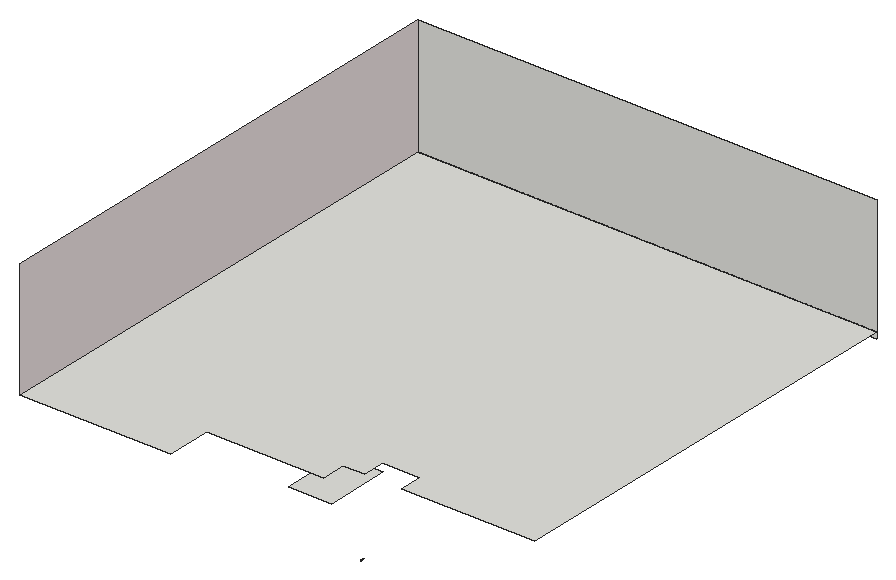
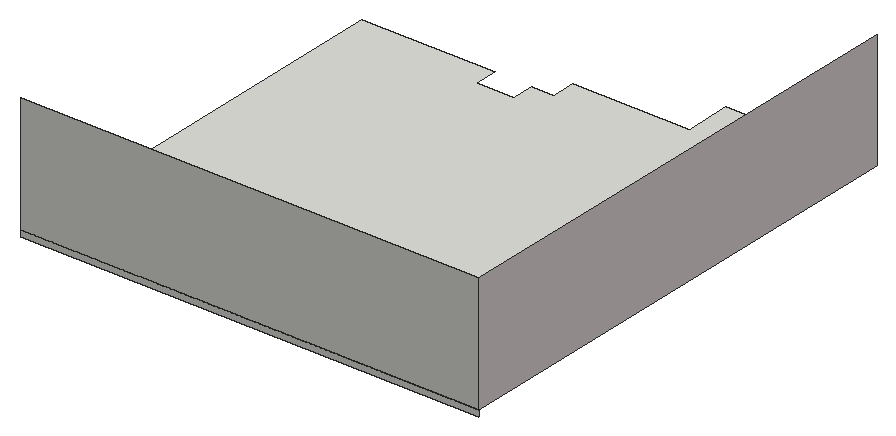
# SketchUp Ruby script. Lengths in inches.
U = 1.inch
M = Sketchup.active_model
def pt(a) = Geom::Point3d.new(a.map { |v| v * U })
def face(e, loops, mat)
  f = e.add_face(loops[0].map { |a| pt(a) })
  loops[1..].each { |l| e.add_face(l.map { |a| pt(a) }).erase! }
  f.material = f.back_material = mat if mat
  f
end
# faces: each face lists its corners as indices into pts; further lists are holes
def faces(e, pts, list, mat = nil) = list.each { |f| face(e, (f[0].is_a?(Array) ? f : [f]).map { |l| l.map { |i| pts[i] } }, mat) }
# xy, xz, yz: faces in a plane at the given z, y or x. An outline is a flat list of corners, or four numbers for a rectangle; further outlines are holes
def ring(l) = l.size == 4 ? [[l[0], l[1]], [l[2], l[1]], [l[2], l[3]], [l[0], l[3]]] : l.each_slice(2).to_a
def flat(e, list, mat, &to3) = list.each { |f| face(e, (f[0].is_a?(Array) ? f : [f]).map { |l| ring(l).map { |u, v| to3.(u, v) } }, mat) }
def xy(e, z, list, mat = nil) = flat(e, list, mat) { |x, y| [x, y, z] }
def xz(e, y, list, mat = nil) = flat(e, list, mat) { |x, z| [x, y, z] }
def yz(e, x, list, mat = nil) = flat(e, list, mat) { |y, z| [x, y, z] }
def lines(e, pts, list) = list.each { |a, b| e.add_line(pt(pts[a]), pt(pts[b])) }
# prism: a flat outline (further loops are holes) pulled along v
def prism(e, loops, v, mat = nil)
  f = face(e, loops, mat); d = Geom::Vector3d.new(v.map { |x| x * U })
  f.pushpull(f.normal.samedirection?(d) ? d.length : -d.length)
end
def box(e, o, s, mat = nil) = prism(e, [[o, [o[0] + s[0], o[1], o[2]], [o[0] + s[0], o[1] + s[1], o[2]], [o[0], o[1] + s[1], o[2]]]], [0, 0, s[2]], mat)
def at(x, y, z, deg = 0) = Geom::Transformation.translation(pt([x, y, z])) * Geom::Transformation.rotation(ORIGIN, Z_AXIS, deg.degrees)
def axes(o, x, y, z) = Geom::Transformation.new([*x, 0, *y, 0, *z, 0, *pt(o).to_a, 1])
def part(name) = M.definitions.add(name)
# library, detail: a bought-in or finely detailed component or shape, given as its bounding box
def library(name, o, s) = part(name).tap { |d| box(d.entities, o, s) }
def detail(e, o, s) = box(e.add_group.entities, o, s)
def put(e, d, t, mat = nil) = e.add_instance(d, t).tap { |i| i.material = mat if mat }
def group(e, t, mat = nil) = e.add_group.tap { |g| g.transformation = t; g.material = mat if mat }.entities
root = M.entities
M.materials.add("Generic\#9").color = [233, 223, 223]
M.materials.add("Material \#1").color = [140, 140, 140]
xy(root,89.4,[[280.76,194.8125,322.26,256.5625]])
xy(root,126,[[75.375,127.4375,220.54,127.4375,220.54,171.4375,333.65,171.4375,333.65,194.75,354.24,194.75,354.24,216.25,390.67,216.25,390.67,194.75,518.6875,194.75,518.6875,607.4375,75.375,607.4375]])
xz(root,199.31,[[347.11,46.74,347.11,46.88,347.12,46.875],[347.82,46.79,347.78,46.8,347.82,46.81],[347.82,46.79,347.82,46.81,347.86,46.8125],[347.82,46.79,347.86,46.8125,347.87,46.8],[347.78,46.8,347.74,46.81,347.78,46.8125],
  [347.78,46.8,347.78,46.8125,347.82,46.81],[347.87,46.8,347.86,46.8125,347.9,46.82],[347.87,46.8,347.9,46.82,347.91,46.81],[347.74,46.81,347.7,46.83,347.74,46.82],[347.74,46.81,347.74,46.82,347.78,46.8125],
  [347.12,46.875,347.11,46.88,347.14,47],[347.12,46.875,347.14,47,347.16,47],[347.14,47,347.2,47.12,347.16,47],[347.625,47.16,347.64,47.2,347.65,47.19],[347.65,47.19,347.64,47.2,347.67,47.23],
  [347.65,47.19,347.67,47.23,347.68,47.22],[347.28,47.22,347.36,47.3125,347.36,47.3],[347.68,47.22,347.67,47.23,347.7,47.25],[347.68,47.22,347.7,47.25,347.71,47.24],[347.71,47.24,347.7,47.25,347.74,47.27],
  [347.71,47.24,347.74,47.27,347.74,47.26],[347.74,47.26,347.74,47.27,347.78,47.28],[347.74,47.26,347.78,47.28,347.78,47.27],[347.36,47.3,347.36,47.3125,347.46,47.39],[347.46,47.375,347.46,47.39,347.57,47.44],
  [347.46,47.375,347.57,47.44,347.58,47.43],[347.58,47.43,347.57,47.44,347.69,47.47],[347.58,47.43,347.69,47.47,347.7,47.46],[347.95,47.46,347.82,47.47,347.95,47.47]],"Material \#1")
xz(root,201.11,[[347.1,46.74,347.11,46.74,347.11,46.88],[347.11,46.74,347.12,46.875,347.11,46.88],[347.82,46.79,347.82,46.81,347.78,46.8],[347.82,46.79,347.86,46.8125,347.82,46.81],[347.82,46.79,347.87,46.8,347.86,46.8125],
  [347.78,46.8,347.78,46.8125,347.74,46.81],[347.78,46.8,347.82,46.81,347.78,46.8125],[347.87,46.8,347.9,46.82,347.86,46.8125],[347.87,46.8,347.91,46.81,347.9,46.82],[347.74,46.81,347.74,46.82,347.7,46.83],
  [347.74,46.81,347.78,46.8125,347.74,46.82],[347.91,46.81,347.9375,46.84,347.9,46.82],[347.74,46.82,347.71,46.84,347.7,46.83],[347.7,46.83,347.71,46.84,347.67,46.85],[347.71,46.84,347.68,46.86,347.67,46.85],
  [347.67,46.85,347.68,46.86,347.64,46.88],[347.68,46.86,347.65,46.89,347.64,46.88],[347.12,46.875,347.14,47,347.11,46.88],[347.12,46.875,347.16,47,347.14,47],[347.64,46.88,347.65,46.89,347.62,46.92],
  [347.65,46.89,347.625,46.92,347.62,46.92],[347.62,46.92,347.625,46.92,347.6,46.95],[347.625,46.92,347.61,46.96,347.6,46.95],[347.6,46.95,347.61,46.96,347.59,47],[347.61,46.96,347.6,47,347.59,47],
  [347.14,47,347.16,47,347.2,47.12],[347.16,47,347.21,47.11,347.2,47.12],[347.59,47,347.6,47,347.58,47.05],[347.6,47,347.6,47.05,347.58,47.05],[347.58,47.05,347.6,47.05,347.59,47.09],
  [347.6,47.05,347.6,47.08,347.59,47.09],[347.6,47.08,347.6,47.13,347.59,47.09],[347.6,47.08,347.61,47.12,347.6,47.13],[347.21,47.11,347.27,47.23,347.2,47.12],[347.21,47.11,347.28,47.22,347.27,47.23],
  [347.61,47.12,347.62,47.17,347.6,47.13],[347.61,47.12,347.625,47.16,347.62,47.17],[347.625,47.16,347.64,47.2,347.62,47.17],[347.625,47.16,347.65,47.19,347.64,47.2],[347.65,47.19,347.67,47.23,347.64,47.2],
  [347.65,47.19,347.68,47.22,347.67,47.23],[347.28,47.22,347.36,47.3125,347.27,47.23],[347.28,47.22,347.36,47.3,347.36,47.3125],[347.68,47.22,347.7,47.25,347.67,47.23],[347.68,47.22,347.71,47.24,347.7,47.25],
  [347.71,47.24,347.74,47.27,347.7,47.25],[347.71,47.24,347.74,47.26,347.74,47.27],[347.95,47.25,347.91,47.27,347.9,47.26],[347.74,47.26,347.78,47.27,347.78,47.28],[347.74,47.26,347.78,47.28,347.74,47.27],
  [347.9,47.26,347.91,47.27,347.86,47.27],[347.78,47.27,347.82,47.28,347.82,47.29],[347.78,47.27,347.82,47.29,347.78,47.28],[347.86,47.27,347.87,47.28,347.82,47.28],[347.86,47.27,347.91,47.27,347.87,47.28],
  [347.82,47.28,347.87,47.28,347.82,47.29],[347.36,47.3,347.46,47.375,347.46,47.39],[347.36,47.3,347.46,47.39,347.36,47.3125],[347.46,47.375,347.57,47.44,347.46,47.39],[347.46,47.375,347.58,47.43,347.57,47.44],
  [347.58,47.43,347.69,47.47,347.57,47.44],[347.58,47.43,347.7,47.46,347.69,47.47],[347.7,47.46,347.82,47.49,347.69,47.47],[347.7,47.46,347.82,47.47,347.82,47.49],[347.95,47.46,347.95,47.47,347.82,47.47],
  [347.82,47.47,347.95,47.47,347.82,47.49]],"Material \#1")
xz(root,607.4375,[[75.375,120,518.6875,126],[75.375,126,518.6875,240]])
yz(root,75.375,[[127.4375,126,607.4375,240]],"Generic\#9")
p = [[347.84,199.31,46.96],[347.84,199.33,46.96],[347.85,199.33,46.93],[347.85,199.31,46.93],[347.87,199.34,46.91],[347.87,199.31,46.91],
  [347.89,199.34,46.92],[347.89,199.31,46.92],[347.92,199.34,46.93],[347.92,199.31,46.93],[347.9,199.33,46.96],[347.9,199.31,46.96],
  [347.84,201.12,46.96],[347.85,201.11,46.93],[347.85,201.09,46.93],[347.84,201.09,46.96],[347.87,201.11,46.91],[347.87,201.08,46.91],
  [347.89,201.11,46.92],[347.89,201.08,46.92],[347.92,201.11,46.93],[347.92,201.08,46.93],[347.9,201.11,46.96],[347.9,201.09,46.96],
  [347.76,199.31,47.09],[347.76,199.33,47.09],[347.89,199.31,46.99],[347.89,199.33,46.99],[347.81,199.33,47.125],[347.81,199.31,47.125],
  [347.76,201.12,47.09],[347.76,201.09,47.09],[347.89,201.12,46.99],[347.81,201.12,47.125],[347.81,201.09,47.125],[347.89,201.09,46.99],
  [347.75,199.31,47.17],[347.75,199.34,47.17],[347.73,199.34,47.15],[347.73,199.31,47.15],[347.75,199.33,47.12],[347.75,199.31,47.12],
  [347.8,199.33,47.15],[347.8,199.31,47.15],[347.78,199.34,47.18],[347.78,199.31,47.18],[347.75,201.11,47.17],[347.73,201.11,47.15],
  [347.73,201.08,47.15],[347.75,201.08,47.17],[347.75,201.11,47.12],[347.75,201.09,47.12],[347.8,201.11,47.15],[347.8,201.09,47.15],
  [347.78,201.11,47.18],[347.78,201.08,47.18]]
faces(root,p,[[0,1,2],[2,3,0],[3,2,4],[4,5,3],[5,4,6],[6,7,5],[7,6,8],[8,9,7],
  [9,8,10],[10,11,9],[12,13,14],[14,15,12],[13,16,17],[17,14,13],[16,18,19],[19,17,16],
  [18,20,21],[21,19,18],[20,22,23],[23,21,20],[24,25,1],[1,0,24],[26,27,28],[28,29,26],
  [11,10,27],[27,26,11],[30,12,15],[15,31,30],[32,33,34],[34,35,32],[22,32,35],[35,23,22],
  [36,37,38],[38,39,36],[39,38,40],[40,41,39],[41,40,25],[25,24,41],[29,28,42],[42,43,29],
  [43,42,44],[44,45,43],[46,47,48],[48,49,46],[47,50,51],[51,48,47],[50,30,31],[31,51,50],
  [33,52,53],[53,34,33],[52,54,55],[55,53,52],[45,44,37],[37,36,45],[54,46,49],[49,55,54]],"Material \#1")
